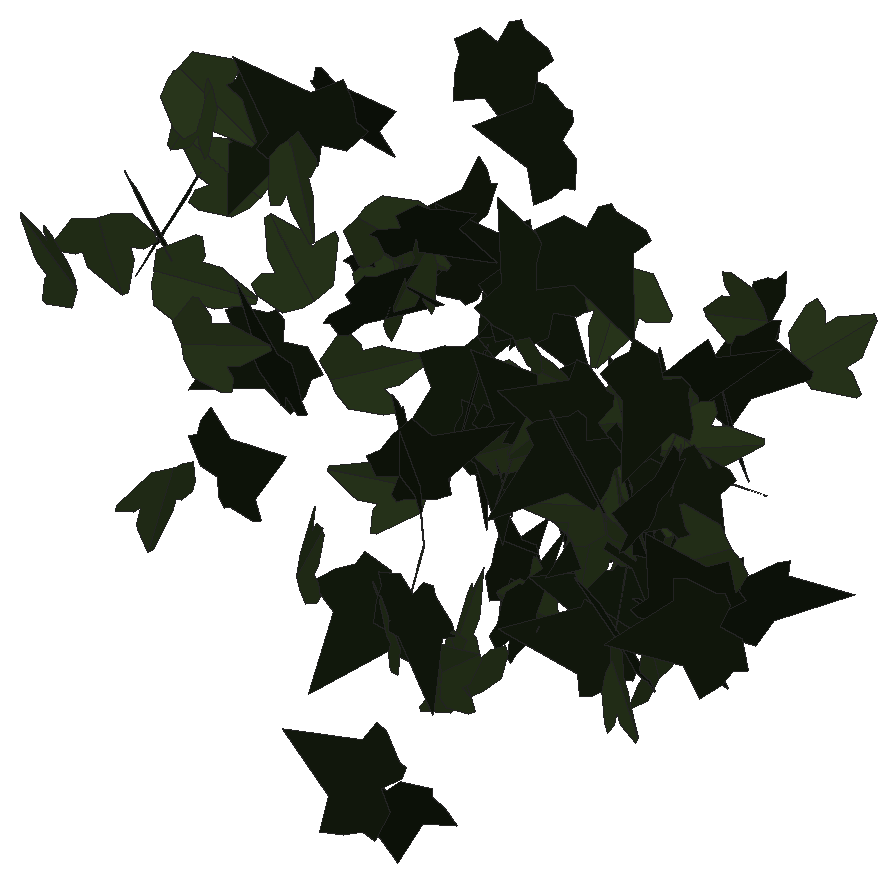
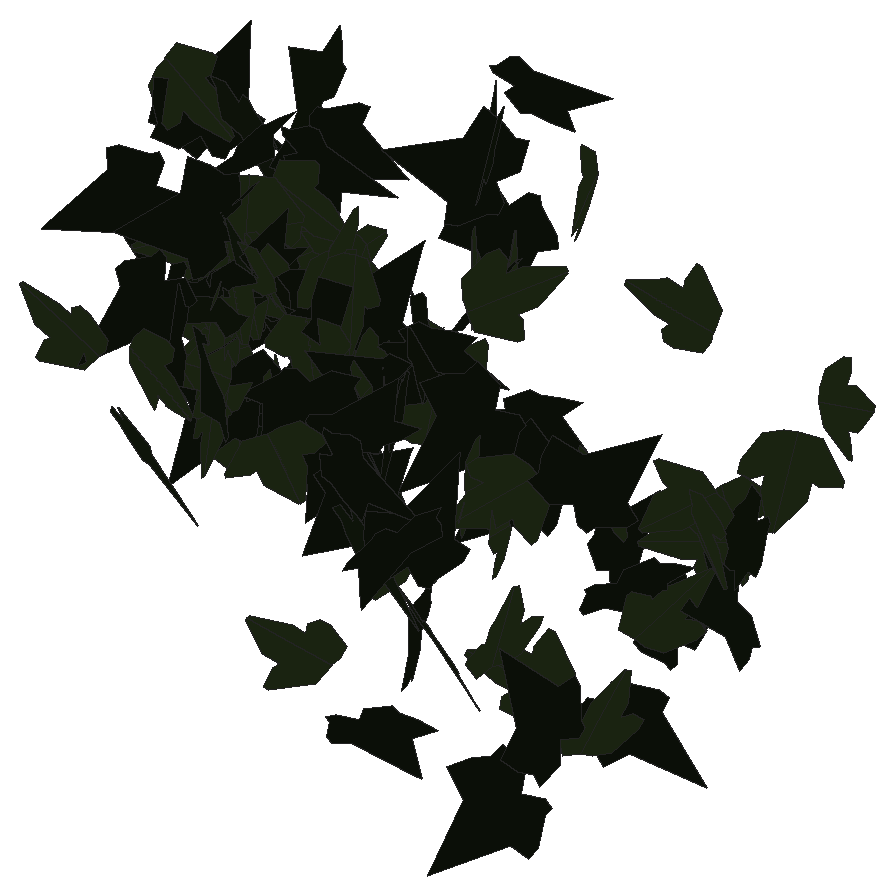
# SketchUp Ruby script. Lengths in inches.
U = 1.inch
M = Sketchup.active_model
def pt(a) = Geom::Point3d.new(a.map { |v| v * U })
def face(e, loops, mat)
  f = e.add_face(loops[0].map { |a| pt(a) })
  loops[1..].each { |l| e.add_face(l.map { |a| pt(a) }).erase! }
  f.material = f.back_material = mat if mat
  f
end
# faces: each face lists its corners as indices into pts; further lists are holes
def faces(e, pts, list, mat = nil) = list.each { |f| face(e, (f[0].is_a?(Array) ? f : [f]).map { |l| l.map { |i| pts[i] } }, mat) }
# xy, xz, yz: faces in a plane at the given z, y or x. An outline is a flat list of corners, or four numbers for a rectangle; further outlines are holes
def ring(l) = l.size == 4 ? [[l[0], l[1]], [l[2], l[1]], [l[2], l[3]], [l[0], l[3]]] : l.each_slice(2).to_a
def flat(e, list, mat, &to3) = list.each { |f| face(e, (f[0].is_a?(Array) ? f : [f]).map { |l| ring(l).map { |u, v| to3.(u, v) } }, mat) }
def xy(e, z, list, mat = nil) = flat(e, list, mat) { |x, y| [x, y, z] }
def xz(e, y, list, mat = nil) = flat(e, list, mat) { |x, z| [x, y, z] }
def yz(e, x, list, mat = nil) = flat(e, list, mat) { |y, z| [x, y, z] }
def lines(e, pts, list) = list.each { |a, b| e.add_line(pt(pts[a]), pt(pts[b])) }
# prism: a flat outline (further loops are holes) pulled along v
def prism(e, loops, v, mat = nil)
  f = face(e, loops, mat); d = Geom::Vector3d.new(v.map { |x| x * U })
  f.pushpull(f.normal.samedirection?(d) ? d.length : -d.length)
end
def box(e, o, s, mat = nil) = prism(e, [[o, [o[0] + s[0], o[1], o[2]], [o[0] + s[0], o[1] + s[1], o[2]], [o[0], o[1] + s[1], o[2]]]], [0, 0, s[2]], mat)
def at(x, y, z, deg = 0) = Geom::Transformation.translation(pt([x, y, z])) * Geom::Transformation.rotation(ORIGIN, Z_AXIS, deg.degrees)
def axes(o, x, y, z) = Geom::Transformation.new([*x, 0, *y, 0, *z, 0, *pt(o).to_a, 1])
def part(name) = M.definitions.add(name)
# library, detail: a bought-in or finely detailed component or shape, given as its bounding box
def library(name, o, s) = part(name).tap { |d| box(d.entities, o, s) }
def detail(e, o, s) = box(e.add_group.entities, o, s)
def put(e, d, t, mat = nil) = e.add_instance(d, t).tap { |i| i.material = mat if mat }
def group(e, t, mat = nil) = e.add_group.tap { |g| g.transformation = t; g.material = mat if mat }.entities
root = M.entities
M.materials.add("efeu1").color = [18, 25, 13]
M.materials.add("efeu2").color = [43, 57, 29]
c1 = part("ivyleaf_9")
p = [[1.54,2.16,1.25],[1.36,2.04,1.19],[-0.21,0.99,0.68],[-0.71,1.11,0.82],[-0.85,0.86,0.67],[-0.8,0.17,0.21],
  [-0.9,-0.01,0.1],[-0.67,-0.16,-0.02],[-0.08,-0.08,-0.05],[-0.03,-0.6,-0.4],[0.65,-0.88,-0.66],[0.83,-0.6,-0.49],
  [1.29,-0.42,-0.43],[1.8125,-0.07,-0.26],[1.21,0.44,0.15]]
faces(c1.entities,p,[[0,1,2,3,4,5,6,7,8,9,10,11,12,13,14]],"efeu1")
c2 = part("ivyleaf_10")
p = [[0,0.5,-0.03],[-0.0625,2.02,-0.43],[-0.19,2.01,-0.46],[-0.54,1.05,-0.29],[-0.52,0.625,-0.18],[-0.83,0.76,-0.28],
  [-1.16,0.64,-0.33],[-1.15,0.33,-0.24],[-0.77,-0.39,0.02],[-0.3,-0.51,0.16],[0.04,-0.48,0.23],[-0.02,2.01,-0.4375],
  [-0.06,2.01,-0.43],[0.04,-0.49,0.23],[0.67,-0.49,0.14],[1.38,0.36,-0.2],[1.375,0.51,-0.24],[0.81,0.65,-0.19],
  [0.62,0.59,-0.15],[0.6,1.09,-0.28],[0.5,1.23,-0.31]]
faces(c2.entities,p,[[0,1,2,3,4,5,6,7,8,9,10],[11,12,0,13,14,15,16,17,18,19,20]],"efeu2")
put(root,c1,axes([37.91,223.35,200.18],[-0.2392,0.35588,-0.25717],[-0.17095,0.19426,0.42783],[0.40443,0.29259,0.02874]))
put(root,c2,axes([37.94,224.08,201.79],[0.38277,-0.23646,-0.21812],[-0.1831,0.11861,-0.44989],[0.2645,0.42429,0.00421]))
put(root,c1,axes([37.54,227.25,200.17],[0.42644,0.0179,-0.26044],[0.25765,0.05148,0.4254],[0.04205,-0.49702,0.03468]))
put(root,c2,axes([38.09,224.72,200.38],[0.14835,0.3428,0.33239],[-0.13053,-0.30569,0.37352],[0.4593,-0.19759,-0.00121]))
put(root,c1,axes([38.04,222.8125,200.97],[0.42283,-0.11273,-0.24189],[-0.23357,0.0629,-0.4376],[0.12909,0.48305,0.00053]))
put(root,c1,axes([38.12,225.29,201.23],[-0.25025,-0.43141,0.03554],[-0.01795,-0.03068,-0.49874],[0.4325,-0.25089,-0.00013]))
put(root,c2,axes([37.84,224.06,201.96],[0.25415,0.14735,0.40459],[0.34967,0.20354,-0.29377],[-0.25128,0.43227,0.00041]))
put(root,c2,axes([38.47,221.56,201.27],[-0.41315,-0.26777,-0.08723],[0.0737,0.04667,-0.49233],[0.2718,-0.41967,0.00091]))
put(root,c2,axes([38.81,220.33,201.3125],[-0.12236,0.10972,-0.47222],[-0.39134,0.26511,0.163],[0.28615,0.40948,0.021]))
put(root,c2,axes([38.55,225.3,198.93],[0.1151,0.46301,0.14959],[-0.04414,-0.14315,0.47703],[0.48457,-0.12302,0.00792]))
put(root,c1,axes([38.58,226.73,198.76],[0.34485,0.3117,0.18417],[0.1327,0.12782,-0.46481],[-0.33685,0.36946,0.00543]))
put(root,c1,axes([39.05,224.23,198.73],[0.03427,0.02867,-0.498],[-0.32969,-0.3733,-0.04418],[-0.37434,0.3314,-0.00668]))
put(root,c2,axes([38.83,222.47,200.33],[0.04465,0.03595,0.4967],[0.39169,0.30544,-0.05732],[-0.30755,0.39423,-0.00089]))
put(root,c1,axes([39.44,224.48,201.5625],[0.11514,0.01372,0.48637],[-0.48273,0.06586,0.11242],[-0.06098,-0.49545,0.02841]))
put(root,c2,axes([39.39,224.01,201.47],[0.3463,-0.09017,0.3492],[0.34369,-0.06422,-0.35742],[0.10931,0.48759,0.01751]))
put(root,c2,axes([40.11,225.14,199.51],[0.04286,0.49789,-0.01642],[-0.01148,0.01747,0.49956],[0.49803,-0.04245,0.01293]))
put(root,c1,axes([40.55,226.02,200.11],[-0.27425,0.31719,0.27236],[-0.1725,0.21086,-0.41926],[-0.38083,-0.32393,-0.00622]))
put(root,c1,axes([40.15,227.08,201.96],[0.0525,-0.44435,-0.22316],[-0.02602,0.22164,-0.44744],[0.49656,0.05859,0.00014]))
put(root,c1,axes([40.52,222.46,199.39],[0.17652,-0.25119,0.39464],[-0.21915,0.32825,0.30696],[-0.4133,-0.28134,0.00579]))
put(root,c1,axes([40.03,221.87,198.31],[-0.00401,0.01259,0.49983],[0.36563,-0.34085,0.01152],[0.34103,0.36559,-0.00647]))
put(root,c2,axes([40.13,224.24,198.64],[-0.16187,-0.1317,0.45437],[0.33877,0.30293,0.20849],[-0.3302,0.37535,-0.00884]))
put(root,c2,axes([40.59,220.13,199.16],[-0.08815,-0.48813,0.06292],[-0.00917,-0.06228,-0.49602],[0.49208,-0.0886,0.00203]))
put(root,c1,axes([40.71,227.02,199.16],[-0.39702,-0.30192,-0.03493],[0.02903,0.01953,-0.49877],[0.30254,-0.39808,0.00202]))
put(root,c2,axes([40.75,223.98,201.08],[-0.2882,-0.09643,-0.39704],[0.37242,0.13785,-0.30381],[0.16806,-0.47085,-0.00763]))
put(root,c2,axes([41.21,223.7,200.21],[0.14629,-0.15537,0.45217],[-0.30352,0.33519,0.21337],[-0.36943,-0.33691,0.00375]))
put(root,c1,axes([41.26,222.93,200.64],[0.25722,0.33562,0.26684],[0.17101,0.20504,-0.42274],[-0.39318,0.30874,-0.00931]))
put(root,c2,axes([41.42,224.09,200.84],[-0.00502,0.12764,-0.48341],[0.02936,-0.48252,-0.12771],[-0.49911,-0.02967,-0.00265]))
put(root,c1,axes([41.58,225.04,200.2],[0.22288,0.14327,0.42403],[-0.38156,-0.18679,0.26367],[0.23396,-0.44112,0.02607]))
put(root,c2,axes([41.26,219.89,201.38],[-0.14803,-0.0404,0.47587],[0.44207,0.17693,0.15254],[-0.18072,0.4659,-0.01666]))
put(root,c1,axes([42.01,225.89,201.85],[-0.1596,-0.05148,-0.47104],[-0.43881,-0.1715,0.16742],[-0.17881,0.46684,0.00956]))
put(root,c1,axes([41.6,223.46,201.5625],[0.38932,0.27388,0.15304],[0.12531,0.08786,-0.476],[-0.28763,0.40899,-0.00023]))
put(root,c1,axes([42.48,224.94,200.33],[-0.36861,0.33649,0.03005],[-0.02428,0.01796,-0.49909],[-0.33695,-0.3694,0.0031]))
put(root,c1,axes([42.19,224.06,198.6],[0.12683,-0.03471,-0.4824],[0.45483,-0.16101,0.13117],[-0.16445,-0.47209,-0.00927]))
put(root,c1,axes([42.5,224.65,200.58],[-0.12261,-0.1213,-0.46931],[0.33315,0.33055,-0.17247],[0.35211,-0.35499,-0.00024]))
put(root,c2,axes([42.63,223.86,199.55],[0.40002,0.18291,0.23776],[0.21578,0.09986,-0.43985],[-0.20839,0.4545,0.00096]))
put(root,c1,axes([43.39,224.01,200.85],[-0.40263,-0.29239,0.04893],[0.04208,0.02531,0.49758],[-0.29345,0.4048,0.00423]))
put(root,c2,axes([43.02,225.0625,198.38],[0.27002,0.12631,-0.40142],[0.3442,0.2081,0.29702],[0.2421,-0.43674,0.02543]))
put(root,c1,axes([43.56,224.52,201.72],[-0.0917,-0.33703,-0.35778],[0.0974,0.34427,-0.34927],[0.48177,-0.13375,0.00252]))
put(root,c2,axes([43.84,224.82,200.93],[0.31344,0.35585,-0.15852],[-0.11229,-0.11229,-0.47411],[-0.37303,0.33281,0.00952]))
put(root,c1,axes([44.1,221.86,200.93],[-0.44052,-0.18724,0.14451],[-0.13213,-0.05854,-0.47866],[0.19617,-0.45991,0.00209]))
put(root,c1,axes([44.03,221.86,201.17],[-0.24235,0.12907,-0.41786],[0.36716,-0.19951,-0.27457],[-0.23761,-0.43993,0.00193]))
put(root,c1,axes([44.28,219.74,199.01],[-0.38269,-0.31117,0.08197],[-0.05918,-0.05714,-0.49319],[0.3163,-0.38718,0.0069]))
put(root,c1,axes([44.26,221.87,200.24],[0.27236,-0.08529,-0.41054],[-0.39002,0.12821,-0.28538],[0.15395,0.4757,0.0033]))
put(root,c2,axes([44.47,219.9375,200.55],[-0.1166,-0.08584,-0.47858],[-0.39543,-0.26962,0.1447],[-0.28291,0.41223,-0.00502]))
put(root,c2,axes([44.59,221.74,200.28],[0.1594,-0.34957,-0.32],[-0.13335,0.29089,-0.38419],[0.45476,0.20782,-0.0005]))
put(root,c1,axes([44.3,221.79,200.39],[0.09675,-0.47303,0.12992],[0.03276,-0.1259,-0.48278],[0.48946,0.10193,0.00663]))
put(root,c1,axes([44.78,221.85,198.48],[0.12113,-0.18409,0.44882],[-0.23801,0.38054,0.22032],[-0.42271,-0.26702,0.00456]))
put(root,c2,axes([44.61,222.03,200.28],[-0.04871,-0.11701,-0.48367],[-0.10116,-0.47351,0.12474],[-0.48723,0.11,0.02246]))
put(root,c1,axes([44.38,221.79,199.99],[-0.06467,-0.02352,0.49524],[0.45955,0.18461,0.06877],[-0.18609,0.46408,-0.00226]))
put(root,c1,axes([44.54,221.66,198.32],[-0.15179,0.3033,0.36738],[0.16495,-0.32827,0.33916],[0.44694,0.22416,-0.0004]))
put(root,c1,axes([44.96,221.91,200.77],[0.17994,0.07187,0.46093],[-0.44258,-0.12987,0.19302],[0.14746,-0.47746,0.01689]))
put(root,c2,axes([45.01,217.29,200.79],[-0.01393,0.00599,0.49977],[-0.32107,0.38305,-0.01354],[-0.38304,-0.3213,-0.00683]))
put(root,c2,axes([45.04,221.87,201.54],[-0.46582,0.10948,0.14501],[-0.14072,0.03506,-0.47851],[-0.11494,-0.48661,-0.00185]))
put(root,c2,axes([45.57,221.25,198.58],[-0.0553,-0.00819,0.49687],[-0.49665,0.0179,-0.05498],[-0.01689,-0.49961,-0.01012]))
put(root,c2,axes([45.36,219.04,200.45],[0.10505,-0.22469,-0.43414],[-0.16282,0.40261,-0.24777],[0.46093,0.19343,0.01142]))
put(root,c1,axes([45.62,225.43,200.83],[-0.4251,0.26324,0.00018],[-0.00018,0.00004,-0.5],[-0.26324,-0.4251,0.00006]))
put(root,c2,axes([45.35,222.23,200.76],[0.49092,0.07805,-0.0539],[-0.07203,0.12189,-0.47953],[-0.06172,0.47859,0.13092]))
put(root,c1,axes([45.31,220.87,198.41],[-0.24221,0.40427,0.16704],[0.07851,-0.14766,0.4712],[0.43032,0.25449,0.00804]))
put(root,c2,axes([45.375,218.48,199.4],[-0.3478,0.28179,0.22278],[0.16435,-0.1509,0.44746],[0.31941,0.38448,0.01234]))
put(root,c1,axes([45.24,219.02,201.65],[-0.00112,-0.12011,0.48536],[0.05795,-0.48212,-0.11918],[0.49663,0.05599,0.015]))
put(root,c2,axes([45.49,221.2,201.31],[-0.41213,0.27686,-0.05914],[0.04917,-0.03287,-0.49649],[-0.2788,-0.41505,-0.00014]))
put(root,c1,axes([45.26,218.85,201.48],[0.10376,0.02119,0.48866],[0.44689,0.19892,-0.10352],[-0.19879,0.45824,0.02235]))
put(root,c2,axes([45.6,221.42,201.21],[-0.19217,-0.45517,-0.07674],[0.03097,0.07022,-0.49408],[0.46056,-0.19464,0.00121]))
put(root,c2,axes([45.63,219.65,198.34],[-0.18739,-0.41687,-0.20275],[-0.08379,-0.18462,0.45705],[-0.45592,0.20527,-0.00066]))
put(root,c1,axes([45.4,218.87,199.79],[0.13128,-0.48057,0.04266],[0.01263,-0.04077,-0.49818],[0.48229,0.13188,0.00144]))
put(root,c2,axes([45.94,224.68,201.3],[0.1677,-0.11094,-0.45778],[-0.39676,0.22864,-0.20076],[0.25388,0.4306,-0.01135]))
put(root,c1,axes([45.28,222.02,198.98],[0.13483,-0.00416,-0.48146],[0.47859,-0.05352,0.13449],[-0.05266,-0.49711,-0.01045]))
put(root,c2,axes([45.58,221.35,201.28],[0.00168,0.00207,0.49999],[0.16605,-0.47162,0.00139],[0.47162,0.16605,-0.00227]))
put(root,c2,axes([45.57,219.61,199.02],[0.34794,-0.34196,-0.10955],[0.07797,-0.07695,0.48785],[-0.35051,-0.35657,-0.00022]))
put(root,c2,axes([45.53,219.16,198.65],[-0.33445,-0.05956,0.36687],[0.36787,0.0174,0.33818],[-0.05305,0.49614,0.03218]))
put(root,c2,axes([46.55,220.73,200.69],[-0.12847,0.02794,0.48241],[-0.46962,-0.1248,-0.11783],[0.11382,-0.48337,0.0583]))
put(root,c2,axes([46.69,221.02,201.74],[-0.16008,-0.04279,0.47174],[-0.44957,-0.14311,-0.16554],[0.14919,-0.47717,0.00734]))
put(root,c2,axes([46.22,221.9,199.28],[0.31834,-0.2923,0.25143],[0.18723,-0.16784,-0.43218],[0.33705,0.36931,0.00259]))
put(root,c1,axes([46.74,221.16,198.625],[-0.25507,-0.01094,0.42991],[-0.42391,-0.07774,-0.25349],[0.07239,-0.4938,0.03038]))
put(root,c1,axes([46.83,220.55,202.01],[-0.2375,-0.10403,-0.42751],[-0.38075,-0.19487,0.25895],[-0.2205,0.44856,0.01334]))
put(root,c2,axes([46.61,220.85,200.3],[-0.46308,-0.09883,0.16059],[-0.1575,-0.03141,-0.47351],[0.10369,-0.48913,-0.00204]))
put(root,c2,axes([46.82,221.67,200.85],[0.00308,0.0199,0.49959],[-0.49181,0.09011,-0.00056],[-0.09006,-0.49141,0.02013]))
put(root,c1,axes([46.9,221.4375,198.99],[-0.17518,0.00792,0.46824],[-0.46811,-0.01735,-0.17484],[0.01348,-0.49964,0.01349]))
put(root,c1,axes([46.82,221.65,201.27],[-0.3655,0.21202,-0.26731],[-0.23518,0.12725,0.42249],[0.24718,0.43458,0.00671]))
put(root,c2,axes([46.79,221.85,201.19],[-0.44258,-0.11628,0.20151],[-0.19521,-0.04998,-0.4576],[0.12656,-0.48372,-0.00116]))
put(root,c1,axes([46.8,221.75,200.82],[-0.27583,-0.38619,0.15741],[0.09034,0.12892,0.47457],[-0.40713,0.29024,-0.00134]))
put(root,c1,axes([46.29,223.58,200.99],[0.07249,0.00026,-0.49472],[0.49114,-0.06007,0.07193],[-0.05939,-0.49638,-0.00897]))
put(root,c1,axes([46.84,222.22,199.61],[-0.00998,0.16856,0.47063],[-0.05329,0.46768,-0.16863],[-0.49705,-0.05353,0.00863]))
put(root,c2,axes([46.69,222.07,201.26],[0.48365,-0.02301,-0.12472],[-0.10995,0.16897,-0.45756],[0.0632,0.47002,0.15839]))
put(root,c1,axes([46.89,221.375,200.42],[0.01879,0.07762,-0.49358],[-0.16012,-0.46694,-0.07953],[-0.4733,0.16105,0.00731]))
put(root,c1,axes([46.89,221.375,201.05],[-0.17561,0.4488,-0.13319],[0.04929,-0.12374,-0.48193],[-0.46555,-0.18239,-0.00078]))
put(root,c1,axes([46.92,221.97,200.49],[-0.47929,-0.11678,0.08148],[0.08039,0.01424,0.49329],[-0.11753,0.48596,0.00512]))
put(root,c2,axes([46.79,221.67,201.93],[-0.39535,-0.30602,-0.00717],[0.00608,0.00385,-0.49995],[0.30605,-0.39539,0.00067]))
put(root,c1,axes([46.79,221.28,198.55],[0.28305,-0.39552,0.11598],[-0.06716,0.09456,0.48636],[-0.40666,-0.2909,0.0004]))
put(root,c1,axes([46.74,223.39,201.5],[0.00047,0.05247,-0.49724],[-0.16174,0.47052,0.04949],[0.47312,0.1608,0.01741]))
put(root,c1,axes([47.02,220.08,201.97],[-0.00157,0.02132,-0.49954],[-0.00071,-0.49955,-0.02131],[-0.5,0.00064,0.0016]))
put(root,c2,axes([46.6,220.77,200.83],[-0.29847,0.05339,-0.39758],[0.39181,-0.06748,-0.3032],[-0.08603,-0.49254,-0.00155]))
put(root,c2,axes([46.95,222.03,199.57],[0.13719,-0.27783,0.39242],[-0.16171,0.35764,0.30974],[-0.4528,-0.2119,0.00828]))
put(root,c2,axes([46.9,221.99,200.6875],[-0.14788,0.18601,0.43992],[0.21954,-0.38252,0.23554],[0.42419,0.26282,0.03146]))
put(root,c1,axes([46.72,221.86,200.89],[0.48547,-0.02296,0.11742],[0.11792,0.17494,-0.45331],[-0.02027,0.46783,0.17527]))
put(root,c1,axes([47.08,221.72,201.46],[0.10379,-0.33788,-0.35365],[0.10188,-0.33866,0.35345],[-0.47838,-0.14543,-0.00145]))
put(root,c2,axes([47.04,221.55,199.98],[0.22796,0.39609,-0.20285],[0.09013,0.1821,0.45685],[0.43579,-0.24486,0.01162]))
put(root,c1,axes([46.89,222.08,201.74],[0.17427,0.13342,0.44925],[0.32943,0.30603,-0.21868],[-0.33333,0.37221,0.01876]))
put(root,c2,axes([47.05,221.92,199.19],[0.05521,-0.48782,-0.09479],[0.11503,0.10533,-0.47505],[0.48345,0.03065,0.12386]))
put(root,c2,axes([47.1,221.57,200.92],[0.189,-0.38309,0.25986],[-0.09916,0.24066,0.42691],[-0.45216,-0.2129,0.015]))
put(root,c2,axes([47.33,220.53,201.07],[-0.34425,0.18388,0.31254],[-0.27822,0.14245,-0.39026],[-0.23257,-0.4426,0.00424]))
put(root,c2,axes([47.13,221.63,199.62],[0.05764,-0.22137,0.4446],[-0.11145,0.43041,0.22875],[-0.484,-0.12548,0.00027]))
put(root,c2,axes([47.11,221.68,200.22],[-0.42884,0.24601,-0.07467],[0.05769,-0.04942,-0.4942],[-0.25053,-0.43248,0.014]))
put(root,c2,axes([46.98,221.5,201.1875],[0.42238,0.21809,0.15502],[0.13817,0.07028,-0.47536],[-0.22913,0.44441,-0.00089]))
put(root,c2,axes([47.11,221.48,198.28],[-0.00957,-0.42157,-0.26867],[-0.01001,-0.2685,0.42167],[-0.49981,0.01345,-0.0033]))
put(root,c2,axes([47.14,221.66,201.17],[0.3631,-0.3402,0.04926],[0.03596,-0.03367,-0.49757],[0.34186,0.36487,0.00002]))
put(root,c2,axes([47.01,221.63,201.12],[0.17264,0.33214,0.33148],[0.12207,0.30926,-0.37344],[-0.45309,0.20987,0.0257]))
put(root,c2,axes([46.89,221.92,200.53],[-0.15109,0.02316,0.47606],[0.47498,-0.03418,0.1524],[0.03961,0.49829,-0.01168]))
put(root,c1,axes([47.02,221.59,199.88],[-0.03478,-0.46997,0.16708],[0.15288,-0.16947,-0.44487],[0.47478,0.02014,0.15549]))
put(root,c1,axes([47.16,221.42,202.27],[-0.09535,-0.45314,0.18859],[-0.0365,-0.18504,-0.46306],[0.48946,-0.10208,0.00221]))
put(root,c1,axes([47.32,215.98,199.06],[0.3204,0.29967,-0.23987],[-0.17636,-0.1626,-0.4387],[-0.34094,0.36573,0.0015]))
put(root,c1,axes([47.01,221.91,199.875],[0.05545,-0.4969,-0.0045],[0.11733,0.01749,-0.48572],[0.48287,0.05281,0.11854]))
put(root,c2,axes([46.95,224.65,201.17],[0.32239,-0.02001,-0.38166],[0.3821,0.00637,0.32243],[-0.00804,-0.49956,0.0194]))
put(root,c1,axes([47.17,221.45,199.07],[0.48176,0.09719,-0.09201],[-0.09104,-0.01399,-0.49144],[-0.0981,0.49026,0.00421]))
put(root,c2,axes([46.97,220.74,198.45],[0.12925,-0.06382,0.47877],[0.44808,-0.16919,-0.14352],[0.18033,0.46616,0.01346]))
put(root,c1,axes([47.19,221.06,200.61],[0.02552,-0.19832,0.45828],[0.0639,-0.45381,-0.19994],[0.49524,0.06878,0.00219]))
put(root,c2,axes([47.13,221.6,199.63],[-0.23445,-0.05452,-0.43825],[0.42837,0.09258,-0.24068],[0.10739,-0.48832,0.0033]))
put(root,c2,axes([47.27,221.6875,201.32],[-0.04818,-0.05223,-0.49492],[0.37094,0.32772,-0.0707],[0.33178,-0.37399,0.00717]))
put(root,c1,axes([47.36,219.53,202.16],[0.14687,-0.27698,0.38951],[0.18695,-0.34172,-0.31349],[0.43986,0.23772,0.00319]))
put(root,c1,axes([47.46,221.33,201.15],[0.06306,-0.41903,-0.2654],[0.07864,0.2726,-0.41171],[0.48973,0.01018,0.10028]))
put(root,c1,axes([48.12,214.76,199.96],[-0.3381,-0.17518,-0.32404],[-0.28932,-0.14596,0.38078],[-0.228,0.44498,-0.00267]))
put(root,c1,axes([48.4,219.78,201.79],[-0.25627,0.40138,0.15237],[-0.08808,0.12453,-0.47617],[-0.4202,-0.27089,0.00688]))
put(root,c2,axes([49.62,219.49,201.66],[-0.25252,-0.0722,0.42547],[-0.41201,-0.10634,-0.26257],[0.1284,-0.4832,-0.00579]))
put(root,c1,axes([49.37,219.3,200.91],[0.28369,0.10071,0.39922],[-0.37514,-0.13657,0.30103],[0.16968,-0.47033,-0.00193]))
put(root,c1,axes([49.36,220.29,200.55],[0.00332,0.21502,-0.45139],[0.02553,0.45074,0.2149],[0.49934,-0.02447,-0.00798]))
put(root,c1,axes([49.96,218.98,200.95],[-0.08507,-0.1092,-0.48046],[-0.32441,-0.35455,0.13802],[-0.37084,0.33522,-0.01053]))
